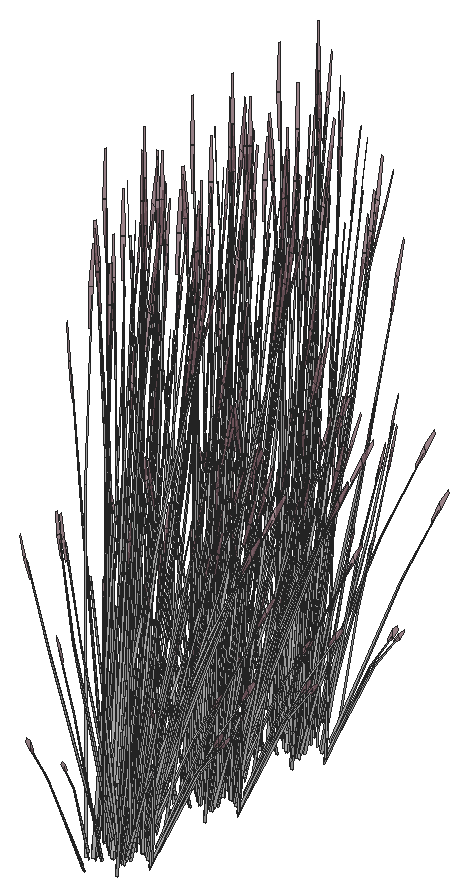
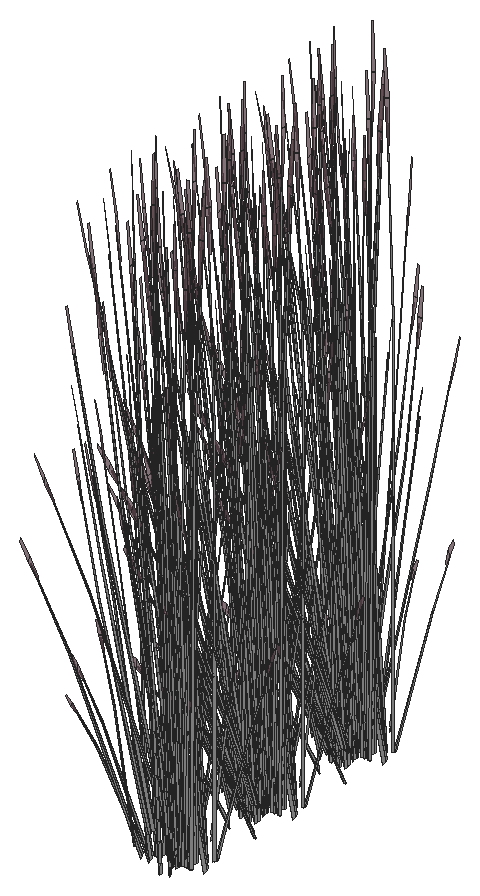
# SketchUp Ruby script. Lengths in inches.
U = 1.inch
M = Sketchup.active_model
def pt(a) = Geom::Point3d.new(a.map { |v| v * U })
def face(e, loops, mat)
  f = e.add_face(loops[0].map { |a| pt(a) })
  loops[1..].each { |l| e.add_face(l.map { |a| pt(a) }).erase! }
  f.material = f.back_material = mat if mat
  f
end
# faces: each face lists its corners as indices into pts; further lists are holes
def faces(e, pts, list, mat = nil) = list.each { |f| face(e, (f[0].is_a?(Array) ? f : [f]).map { |l| l.map { |i| pts[i] } }, mat) }
# xy, xz, yz: faces in a plane at the given z, y or x. An outline is a flat list of corners, or four numbers for a rectangle; further outlines are holes
def ring(l) = l.size == 4 ? [[l[0], l[1]], [l[2], l[1]], [l[2], l[3]], [l[0], l[3]]] : l.each_slice(2).to_a
def flat(e, list, mat, &to3) = list.each { |f| face(e, (f[0].is_a?(Array) ? f : [f]).map { |l| ring(l).map { |u, v| to3.(u, v) } }, mat) }
def xy(e, z, list, mat = nil) = flat(e, list, mat) { |x, y| [x, y, z] }
def xz(e, y, list, mat = nil) = flat(e, list, mat) { |x, z| [x, y, z] }
def yz(e, x, list, mat = nil) = flat(e, list, mat) { |y, z| [x, y, z] }
def lines(e, pts, list) = list.each { |a, b| e.add_line(pt(pts[a]), pt(pts[b])) }
# prism: a flat outline (further loops are holes) pulled along v
def prism(e, loops, v, mat = nil)
  f = face(e, loops, mat); d = Geom::Vector3d.new(v.map { |x| x * U })
  f.pushpull(f.normal.samedirection?(d) ? d.length : -d.length)
end
def box(e, o, s, mat = nil) = prism(e, [[o, [o[0] + s[0], o[1], o[2]], [o[0] + s[0], o[1] + s[1], o[2]], [o[0], o[1] + s[1], o[2]]]], [0, 0, s[2]], mat)
def at(x, y, z, deg = 0) = Geom::Transformation.translation(pt([x, y, z])) * Geom::Transformation.rotation(ORIGIN, Z_AXIS, deg.degrees)
def axes(o, x, y, z) = Geom::Transformation.new([*x, 0, *y, 0, *z, 0, *pt(o).to_a, 1])
def part(name) = M.definitions.add(name)
# library, detail: a bought-in or finely detailed component or shape, given as its bounding box
def library(name, o, s) = part(name).tap { |d| box(d.entities, o, s) }
def detail(e, o, s) = box(e.add_group.entities, o, s)
def put(e, d, t, mat = nil) = e.add_instance(d, t).tap { |i| i.material = mat if mat }
def group(e, t, mat = nil) = e.add_group.tap { |g| g.transformation = t; g.material = mat if mat }.entities
root = M.entities
M.materials.add("LightPink_Translucent").color = [144, 107, 117]
M.materials["LightPink_Translucent"].alpha = 0.75
M.materials.add("[_0053_Ivory_]").color = [200, 200, 200]
c1 = part("blade")
p = [[2.15,0.21,22],[0,0.17,0],[0.09,0.45,0],[2.18,0.31,22],[2.29,0.31,22],[0.38,0.45,0],
  [2.48,0.24,33],[2.49,0.24,33],[2.48,0.22,33]]
faces(c1.entities,p,[[0,1,2,3],[4,5,2,3],[6,3,4,7],[8,0,3,6]])
c2 = part("seeds")
p = [[0.3,-0.1,1.38],[-0.01,-0.03,1.59],[-0.01,-0.03,0.03],[0.14,-0.07,-0.07],[0.29,-0.03,3],[0.15,0.01,3.11]]
faces(c2.entities,p,[[0,1,2,3],[1,0,4,5]],"LightPink_Translucent")
c3 = part("blade with seeds")
put(c3.entities,c1,at(0,0,0))
put(c3.entities,c2,axes([2.4,0.25,30.99],[1.5799,-0.05474,1.17369],[-0.12525,1.92788,0.29478],[-0.07173,-0.02425,1.56792]))
put(root,c3,axes([680.98,251.57,36.24],[-0.17264,0.12729,1.43002],[-0.51703,-0.22279,-0.30754],[0.09584,-0.27707,0.61141]),"[_0053_Ivory_]")
put(root,c3,axes([679.7,250.88,35.15],[-0.10187,0.02266,1.76342],[-0.56336,-0.25503,-0.26939],[0.00945,-0.21273,0.30037]),"[_0053_Ivory_]")
put(root,c3,axes([681.4,252.52,38.63],[0.0158,-0.58168,-0.71045],[0.66548,0.03907,0.08574],[0.07023,-0.24643,1.00501]),"[_0053_Ivory_]")
put(root,c3,axes([680.25,251.58,38.18],[0.1831,-0.48359,-0.35414],[0.53419,0.14105,0.4572],[-0.04898,-0.1947,0.87481]),"[_0053_Ivory_]")
put(root,c3,axes([680.65,252.22,37.53],[-0.11309,0.21615,1.71376],[-0.47441,-0.44731,0.13857],[0.21402,-0.27879,0.73262]),"[_0053_Ivory_]")
put(root,c3,axes([680.35,250.5625,36.42],[0.07791,0.3667,1.1486],[-0.43222,-0.2031,0.84392],[0.04651,-0.18776,0.25299]),"[_0053_Ivory_]")
put(root,c3,axes([681.27,252.32,38.33],[-0.43478,-0.42253,-0.51099],[0.45929,-0.37004,-0.3958],[0.06615,-0.21468,0.97773]),"[_0053_Ivory_]")
put(root,c3,axes([681.68,252.17,38.18],[0.41095,-0.33109,-0.35414],[0.38901,0.37805,0.4572],[0.05919,-0.19208,0.87481]),"[_0053_Ivory_]")
put(root,c3,axes([682.19,251.97,35.15],[-0.0909,-0.04954,1.76342],[-0.2335,-0.55347,-0.26939],[0.15752,-0.1502,0.30037]),"[_0053_Ivory_]")
put(root,c3,axes([682.1875,253.53,38.63],[0.31725,-0.49618,-0.71045],[0.55593,0.35263,0.08574],[0.18942,-0.17977,1.00501]),"[_0053_Ivory_]")
put(root,c3,axes([678.76,252.08,36.03],[-0.37973,-0.63014,0],[0.6353,-0.35142,-0.51607],[0.14469,-0.08004,1.63711]),"[_0053_Ivory_]")
put(root,c3,axes([682.17,253.3,38.33],[-0.15602,-0.5742,-0.51099],[0.59087,-0.10045,-0.3958],[0.16933,-0.15423,0.97773]),"[_0053_Ivory_]")
put(root,c3,axes([679.27,251.99,35.67],[0.56842,-0.31443,-0.49651],[0.33976,0.56381,0],[0.12946,-0.07161,1.57504]),"[_0053_Ivory_]")
put(root,c3,axes([682.65,253.07,36.24],[-0.21697,-0.01863,1.43002],[-0.22228,-0.49966,-0.30754],[0.26655,-0.14135,0.61141]),"[_0053_Ivory_]")
put(root,c3,axes([679.95,253.28,35.71],[0.40909,-0.47266,-0.62353],[0.50819,0.4286,-0.16365],[0.16393,-0.11791,1.37633]),"[_0053_Ivory_]")
put(root,c3,axes([682.9,252.15,36.42],[-0.2023,0.32011,1.1486],[-0.17388,-0.43009,0.84392],[0.16708,-0.10777,0.25299]),"[_0053_Ivory_]")
put(root,c3,axes([682.61,253.36,38.18],[0.52868,-0.08987,-0.35414],[0.1396,0.51376,0.4572],[0.1515,-0.13799,0.87481]),"[_0053_Ivory_]")
put(root,c3,axes([679.24,254.1,35.86],[0.29468,-0.56664,-0.44739],[0.61229,0.27271,0.21531],[0,-0.13062,1.43643]),"[_0053_Ivory_]")
put(root,c3,axes([679.5,253.82,36.32],[-0.07077,-0.71755,-0.29095],[0.73712,-0.04339,-0.50002],[0.1298,-0.09558,1.59708]),"[_0053_Ivory_]")
put(root,c3,axes([679.41,252.23,35.68],[0.56663,0.1556,-0.30978],[-0.14267,0.54795,0.30978],[0.11423,-0.06319,1.38974]),"[_0053_Ivory_]")
put(root,c3,axes([679.6,254.39,36.09],[0.68433,0.30479,0.24065],[-0.32934,0.63331,0.50002],[0,-0.14599,1.60543]),"[_0053_Ivory_]")
put(root,c3,axes([679.38,253.96,36.37],[-0.65953,0.03882,0.44739],[-0.05964,-0.64439,-0.21531],[0.11807,-0.06531,1.43643]),"[_0053_Ivory_]")
put(root,c3,axes([682.45,254.57,38.33],[0.16454,-0.57202,-0.51099],[0.56413,0.19607,-0.3958],[0.22713,-0.05245,0.97773]),"[_0053_Ivory_]")
put(root,c3,axes([681.55,252.24,36.03],[0.37973,-0.63014,0],[0.6353,0.35142,-0.51607],[0.14469,0.08004,1.63711]),"[_0053_Ivory_]")
put(root,c3,axes([679.36,254.19,36.01],[0.26406,0.70318,0.45755],[-0.7545,0.24452,0.17955],[0.00922,-0.12921,1.58856]),"[_0053_Ivory_]")
put(root,c3,axes([683.05,254.73,35.64],[-0.39118,0.07547,1.41583],[-0.06226,-0.6007,0.08104],[0.27398,-0.09092,0.80566]),"[_0053_Ivory_]")
put(root,c3,axes([683.76,254.2,35.91],[-0.37654,-0.40212,-0.06488],[0.4124,-0.36845,-0.29416],[0.11685,-0.02594,0.97024]),"[_0053_Ivory_]")
put(root,c3,axes([680.31,254.25,35.86],[0,-0.72763,0],[0.75945,0,0],[0,0,1.79456]),"[_0053_Ivory_]")
put(root,c3,axes([681.23,252.57,36.13],[-0.56842,-0.31443,0.49651],[0.33976,-0.56381,0],[0.12946,0.07161,1.57504]),"[_0053_Ivory_]")
put(root,c3,axes([682.34,254.78,38.63],[0.53369,-0.27773,-0.71045],[0.29743,0.5717,0.08574],[0.25786,-0.06494,1.00501]),"[_0053_Ivory_]")
put(root,c3,axes([679.95,253.79,36.01],[-0.50358,0.57069,0.45755],[-0.59827,-0.50377,0.17955],[0.1214,-0.05695,1.58856]),"[_0053_Ivory_]")
put(root,c3,axes([679.07,252.85,36.13],[-0.17545,0.62497,0.17642],[-0.64204,-0.17686,0.35086],[0.11091,-0.00304,1.60407]),"[_0053_Ivory_]")
put(root,c3,axes([678.81,253.36,35.25],[-0.59782,0.25177,1.28929],[-0.19028,-0.72239,0.50096],[0.36709,0.01202,1.46642]),"[_0053_Ivory_]")
put(root,c3,axes([680.41,253.55,36.27],[0.11717,-0.56122,0.1448],[0.57245,0.09742,-0.41347],[0.10418,0.05763,1.26744]),"[_0053_Ivory_]")
put(root,c3,axes([683.48,254.34,35.15],[-0.03174,-0.09547,1.76342],[0.22015,-0.55846,-0.26939],[0.22208,-0.00803,0.30037]),"[_0053_Ivory_]")
put(root,c3,axes([680.17,253.7,36.37],[-0.36485,-0.52782,0.44739],[0.55265,-0.37168,-0.21531],[0.11807,0.06531,1.43643]),"[_0053_Ivory_]")
put(root,c3,axes([680.35,253.73,36.32],[0.61322,-0.4175,-0.29095],[0.40778,0.58992,-0.50002],[0.1513,0.05991,1.59708]),"[_0053_Ivory_]")
put(root,c3,axes([682.79,254.83,38.18],[0.50475,0.17543,-0.35414],[-0.14722,0.5118,0.4572],[0.20322,-0.04693,0.87481]),"[_0053_Ivory_]")
put(root,c3,axes([681.9,252.62,35.67],[0.56842,0.31443,-0.49651],[-0.33976,0.56381,0],[0.12946,0.07161,1.57504]),"[_0053_Ivory_]")
put(root,c3,axes([680.82,254.42,35.86],[0.67951,0,0],[0,0.65103,0],[0,0,1.78407]),"[_0053_Ivory_]")
put(root,c3,axes([681.01,252.89,36.13],[-0.65264,0.16691,0.17642],[-0.16115,-0.62115,0.35086],[0.05821,0.0905,1.60407]),"[_0053_Ivory_]")
put(root,c3,axes([681.42,254.2,37.53],[-0.25192,0.01424,1.71376],[0.16712,-0.61729,0.13857],[0.35901,0.03818,0.73262]),"[_0053_Ivory_]")
put(root,c3,axes([681.74,252.86,35.68],[0.14267,0.54795,-0.30978],[-0.56663,0.1556,0.30978],[0.11423,0.06319,1.38974]),"[_0053_Ivory_]")
put(root,c3,axes([680.6,254.08,36.03],[-0.76764,-0.13249,0.49198],[0.15622,-0.74829,0.19306],[0.11218,0.07226,1.70813]),"[_0053_Ivory_]")
put(root,c3,axes([679.99,255.93,35.86],[-0.19817,-0.54216,0],[0.56587,-0.18986,0],[0,0,1.54371]),"[_0053_Ivory_]")
put(root,c3,axes([680.73,255.86,35.84],[0.63764,-0.21337,-0.19198],[0.22406,0.61462,0.00008],[0.07038,-0.02358,1.73897]),"[_0053_Ivory_]")
put(root,c3,axes([680.81,254.69,35.87],[0.42396,0.40619,0],[-0.42396,0.40619,0],[0,0,1.69266]),"[_0053_Ivory_]")
put(root,c3,axes([681.95,254.52,36.13],[-0.47719,-0.45806,0.17642],[0.48088,-0.44429,0.35086],[-0.0527,0.09355,1.60407]),"[_0053_Ivory_]")
put(root,c3,axes([681.07,253.83,35.71],[0.63179,0.1031,-0.62353],[-0.13332,0.63596,-0.16365],[0.18854,0.07706,1.37633]),"[_0053_Ivory_]")
put(root,c3,axes([683.86,254.9375,36.42],[-0.37526,0.10382,1.1486],[0.17664,-0.42906,0.84392],[0.19907,0.02936,0.25299]),"[_0053_Ivory_]")
put(root,c3,axes([680.8,254.22,36.37],[0.29468,-0.56664,0.44739],[0.61229,0.27271,-0.21531],[0,0.13062,1.43643]),"[_0053_Ivory_]")
put(root,c3,axes([680.6875,254.54,35.95],[0,0.72727,-0.05637],[-0.75945,0,0],[0,0.02286,1.79368]),"[_0053_Ivory_]")
put(root,c3,axes([680.74,254.03,35.86],[0.36485,0.52782,-0.44739],[-0.55265,0.37168,0.21531],[0.11807,0.06531,1.43643]),"[_0053_Ivory_]")
put(root,c3,axes([683.21,256.26,37.58],[-0.11624,-0.52862,-0.03492],[0.54943,-0.12153,-0.15832],[0.11473,0.03351,0.52218]),"[_0053_Ivory_]")
put(root,c3,axes([682.35,254.54,36.13],[0,-0.62885,0.49651],[0.67951,0,0],[0,0.14322,1.57504]),"[_0053_Ivory_]")
put(root,c3,axes([681.06,254.35,36.27],[0.56587,-0.18339,0.1448],[0.19817,0.52368,-0.41347],[0,0.11525,1.26744]),"[_0053_Ivory_]")
put(root,c3,axes([683.16,255.625,36.24],[-0.14627,-0.15466,1.43002],[0.19032,-0.51164,-0.30754],[0.29594,0.06931,0.61141]),"[_0053_Ivory_]")
put(root,c3,axes([680.55,256.1875,35.86],[0.61229,0.28233,0],[-0.29468,0.58663,0],[0,0,1.74954]),"[_0053_Ivory_]")
put(root,c3,axes([681.82,255.9375,38.63],[0.60713,0.01514,-0.71045],[-0.04078,0.63759,0.08574],[0.25721,0.06729,1.00501]),"[_0053_Ivory_]")
put(root,c3,axes([681.13,256.45,36.13],[0.56842,-0.31443,0.49651],[0.33976,0.56381,0],[-0.12946,0.07161,1.57504]),"[_0053_Ivory_]")
put(root,c3,axes([680.32,255.95,35.94],[0.26406,0.72244,-0.06012],[-0.7545,0.25315,0],[0.00922,0.02523,1.72173]),"[_0053_Ivory_]")
put(root,c3,axes([682.81,254.64,36.03],[0.75945,0,0],[0,0.70283,-0.51607],[0,0.16007,1.63711]),"[_0053_Ivory_]")
put(root,c3,axes([682.51,255,35.85],[-0.75908,-0.00503,-0.04976],[0,-0.70283,0.49943],[-0.02386,0.16,1.58352]),"[_0053_Ivory_]")
put(root,c3,axes([680.86,254.39,36.32],[0.68399,0.30005,-0.29095],[-0.32934,0.63331,-0.50002],[0.0215,0.15549,1.59708]),"[_0053_Ivory_]")
put(root,c3,axes([680.98,262.72,36.24],[-0.17264,0.12729,1.43002],[-0.51703,-0.22279,-0.30754],[0.09584,-0.27707,0.61141]),"[_0053_Ivory_]")
put(root,c3,axes([682.18,256.2,38.18],[0.34557,0.39372,-0.35414],[-0.39459,0.37271,0.4572],[0.20048,0.05671,0.87481]),"[_0053_Ivory_]")
put(root,c3,axes([682.35,255.11,35.68],[-0.42396,0.39235,-0.30978],[-0.42396,-0.39235,0.30978],[0,0.12637,1.38974]),"[_0053_Ivory_]")
put(root,c3,axes([680.79,254.86,35.86],[-0.29468,0.56664,-0.44739],[-0.61229,-0.27271,0.21531],[0,0.13062,1.43643]),"[_0053_Ivory_]")
put(root,c3,axes([679.7,262.03,35.15],[-0.10187,0.02266,1.76342],[-0.56336,-0.25503,-0.26939],[0.00945,-0.21273,0.30037]),"[_0053_Ivory_]")
put(root,c3,axes([681.4,263.67,38.63],[0.0158,-0.58168,-0.71045],[0.66548,0.03907,0.08574],[0.07023,-0.24643,1.00501]),"[_0053_Ivory_]")
put(root,c3,axes([680.25,262.73,38.18],[0.1831,-0.48359,-0.35414],[0.53419,0.14105,0.4572],[-0.04898,-0.1947,0.87481]),"[_0053_Ivory_]")
put(root,c3,axes([680.65,263.37,37.53],[-0.11309,0.21615,1.71376],[-0.47441,-0.44731,0.13857],[0.21402,-0.27879,0.73262]),"[_0053_Ivory_]")
put(root,c3,axes([682.64,255.12,35.67],[0,0.62885,-0.49651],[-0.67951,0,0],[0,0.14322,1.57504]),"[_0053_Ivory_]")
put(root,c3,axes([680.94,255.19,37.53],[-0.2256,-0.10835,1.71376],[0.46687,-0.45453,0.13857],[0.29098,0.20505,0.73262]),"[_0053_Ivory_]")
put(root,c3,axes([680.35,261.71,36.42],[0.07791,0.3667,1.1486],[-0.43222,-0.2031,0.84392],[0.04651,-0.18776,0.25299]),"[_0053_Ivory_]")
put(root,c3,axes([681.27,263.47,38.33],[-0.43478,-0.42253,-0.51099],[0.45929,-0.37004,-0.3958],[0.06615,-0.21468,0.97773]),"[_0053_Ivory_]")
put(root,c3,axes([681.78,256.42,36.42],[-0.34197,-0.18082,1.1486],[0.44156,-0.18372,0.84392],[0.1191,0.15563,0.25299]),"[_0053_Ivory_]")
put(root,c3,axes([681.87,257.1,35.15],[0.04425,-0.09079,1.76342],[0.55709,-0.26738,-0.26939],[0.16889,0.13839,0.30037]),"[_0053_Ivory_]")
put(root,c3,axes([681.14,255.03,35.75],[0.2227,0.57576,-0.69212],[-0.64151,0.20736,-0.18165],[0.02462,0.19497,1.52773]),"[_0053_Ivory_]")
put(root,c3,axes([681.68,263.32,38.18],[0.41095,-0.33109,-0.35414],[0.38901,0.37805,0.4572],[0.05919,-0.19208,0.87481]),"[_0053_Ivory_]")
put(root,c3,axes([681,256.67,38.33],[0.59932,-0.14948,-0.51099],[0.10484,0.56611,-0.3958],[0.16097,0.16223,0.97773]),"[_0053_Ivory_]")
put(root,c3,axes([681.83,257.25,36.32],[-0.38947,-0.01972,1.0506],[0.25721,-0.41888,0.58006],[0.15386,0.14882,0.8241]),"[_0053_Ivory_]")
put(root,c3,axes([682.19,263.12,35.15],[-0.0909,-0.04954,1.76342],[-0.2335,-0.55347,-0.26939],[0.15752,-0.1502,0.30037]),"[_0053_Ivory_]")
put(root,c3,axes([680.56,256.23,36.24],[0.01072,-0.20846,1.43002],[0.51218,-0.23285,-0.30754],[0.15811,0.2495,0.61141]),"[_0053_Ivory_]")
put(root,c3,axes([682.1875,264.68,38.63],[0.31725,-0.49618,-0.71045],[0.55593,0.35263,0.08574],[0.18942,-0.17977,1.00501]),"[_0053_Ivory_]")
put(root,c3,axes([678.76,263.23,36.03],[-0.37973,-0.63014,0],[0.6353,-0.35142,-0.51607],[0.14469,-0.08004,1.63711]),"[_0053_Ivory_]")
put(root,c3,axes([682.17,264.44,38.33],[-0.15602,-0.5742,-0.51099],[0.59087,-0.10045,-0.3958],[0.16933,-0.15423,0.97773]),"[_0053_Ivory_]")
put(root,c3,axes([679.27,257.08,35.15],[0.09829,-0.03422,1.76342],[0.59126,0.18834,-0.26939],[0.01729,0.21228,0.30037]),"[_0053_Ivory_]")
put(root,c3,axes([679.67,256.94,38.33],[0.59704,0.15764,-0.51099],[-0.20464,0.54049,-0.3958],[0.05475,0.21761,0.97773]),"[_0053_Ivory_]")
put(root,c3,axes([680.01,255.82,37.53],[-0.13883,-0.2019,1.71376],[0.64153,-0.16998,0.13857],[0.14499,0.31697,0.73262]),"[_0053_Ivory_]")
put(root,c3,axes([679.4,257.27,38.18],[-0.1831,0.48359,-0.35414],[-0.53419,-0.14105,0.4572],[0.04898,0.1947,0.87481]),"[_0053_Ivory_]")
put(root,c3,axes([679.27,263.13,35.67],[0.56842,-0.31443,-0.49651],[0.33976,0.56381,0],[0.12946,-0.07161,1.57504]),"[_0053_Ivory_]")
put(root,c3,axes([682.65,264.22,36.24],[-0.21697,-0.01863,1.43002],[-0.22228,-0.49966,-0.30754],[0.26655,-0.14135,0.61141]),"[_0053_Ivory_]")
put(root,c3,axes([679.95,264.42,35.71],[0.40909,-0.47266,-0.62353],[0.50819,0.4286,-0.16365],[0.16393,-0.11791,1.37633]),"[_0053_Ivory_]")
put(root,c3,axes([682.9,263.3,36.42],[-0.2023,0.32011,1.1486],[-0.17388,-0.43009,0.84392],[0.16708,-0.10777,0.25299]),"[_0053_Ivory_]")
put(root,c3,axes([682.61,264.51,38.18],[0.52868,-0.08987,-0.35414],[0.1396,0.51376,0.4572],[0.1515,-0.13799,0.87481]),"[_0053_Ivory_]")
put(root,c3,axes([679.46,256.83,38.63],[0.28988,0.51132,-0.71045],[-0.59671,0.28496,0.08574],[0.06778,0.24706,1.00501]),"[_0053_Ivory_]")
put(root,c3,axes([679.24,265.25,35.86],[0.29468,-0.56664,-0.44739],[0.61229,0.27271,0.21531],[0,-0.13062,1.43643]),"[_0053_Ivory_]")
put(root,c3,axes([679.5,264.97,36.32],[-0.07077,-0.71755,-0.29095],[0.73712,-0.04339,-0.50002],[0.1298,-0.09558,1.59708]),"[_0053_Ivory_]")
put(root,c3,axes([679.41,263.38,35.68],[0.56663,0.1556,-0.30978],[-0.14267,0.54795,0.30978],[0.11423,-0.06319,1.38974]),"[_0053_Ivory_]")
put(root,c3,axes([679.6,265.53,36.09],[0.68433,0.30479,0.24065],[-0.32934,0.63331,0.50002],[0,-0.14599,1.60543]),"[_0053_Ivory_]")
put(root,c3,axes([679.38,265.11,36.37],[-0.65953,0.03882,0.44739],[-0.05964,-0.64439,-0.21531],[0.11807,-0.06531,1.43643]),"[_0053_Ivory_]")
put(root,c3,axes([682.45,265.72,38.33],[0.16454,-0.57202,-0.51099],[0.56413,0.19607,-0.3958],[0.22713,-0.05245,0.97773]),"[_0053_Ivory_]")
put(root,c3,axes([681.55,263.39,36.03],[0.37973,-0.63014,0],[0.6353,0.35142,-0.51607],[0.14469,0.08004,1.63711]),"[_0053_Ivory_]")
put(root,c3,axes([679.36,265.34,36.01],[0.26406,0.70318,0.45755],[-0.7545,0.24452,0.17955],[0.00922,-0.12921,1.58856]),"[_0053_Ivory_]")
put(root,c3,axes([683.05,265.88,35.64],[-0.39118,0.07547,1.41583],[-0.06226,-0.6007,0.08104],[0.27398,-0.09092,0.80566]),"[_0053_Ivory_]")
put(root,c3,axes([683.76,265.35,35.91],[-0.37654,-0.40212,-0.06488],[0.4124,-0.36845,-0.29416],[0.11685,-0.02594,0.97024]),"[_0053_Ivory_]")
put(root,c3,axes([680.31,265.4,35.86],[0,-0.72763,0],[0.75945,0,0],[0,0,1.79456]),"[_0053_Ivory_]")
put(root,c3,axes([681.23,263.72,36.13],[-0.56842,-0.31443,0.49651],[0.33976,-0.56381,0],[0.12946,0.07161,1.57504]),"[_0053_Ivory_]")
put(root,c3,axes([682.34,265.93,38.63],[0.53369,-0.27773,-0.71045],[0.29743,0.5717,0.08574],[0.25786,-0.06494,1.00501]),"[_0053_Ivory_]")
put(root,c3,axes([679.95,264.94,36.01],[-0.50358,0.57069,0.45755],[-0.59827,-0.50377,0.17955],[0.1214,-0.05695,1.58856]),"[_0053_Ivory_]")
put(root,c3,axes([679.07,264,36.13],[-0.17545,0.62497,0.17642],[-0.64204,-0.17686,0.35086],[0.11091,-0.00304,1.60407]),"[_0053_Ivory_]")
put(root,c3,axes([678.81,264.51,35.25],[-0.59782,0.25177,1.28929],[-0.19028,-0.72239,0.50096],[0.36709,0.01202,1.46642]),"[_0053_Ivory_]")
put(root,c3,axes([680.41,264.7,36.27],[0.11717,-0.56122,0.1448],[0.57245,0.09742,-0.41347],[0.10418,0.05763,1.26744]),"[_0053_Ivory_]")
put(root,c3,axes([683.48,265.49,35.15],[-0.03174,-0.09547,1.76342],[0.22015,-0.55846,-0.26939],[0.22208,-0.00803,0.30037]),"[_0053_Ivory_]")
put(root,c3,axes([680.17,264.85,36.37],[-0.36485,-0.52782,0.44739],[0.55265,-0.37168,-0.21531],[0.11807,0.06531,1.43643]),"[_0053_Ivory_]")
put(root,c3,axes([680.35,264.88,36.32],[0.61322,-0.4175,-0.29095],[0.40778,0.58992,-0.50002],[0.1513,0.05991,1.59708]),"[_0053_Ivory_]")
put(root,c3,axes([682.79,265.98,38.18],[0.50475,0.17543,-0.35414],[-0.14722,0.5118,0.4572],[0.20322,-0.04693,0.87481]),"[_0053_Ivory_]")
put(root,c3,axes([681.9,263.77,35.67],[0.56842,0.31443,-0.49651],[-0.33976,0.56381,0],[0.12946,0.07161,1.57504]),"[_0053_Ivory_]")
put(root,c3,axes([680.82,265.5625,35.86],[0.67951,0,0],[0,0.65103,0],[0,0,1.78407]),"[_0053_Ivory_]")
put(root,c3,axes([681.01,264.04,36.13],[-0.65264,0.16691,0.17642],[-0.16115,-0.62115,0.35086],[0.05821,0.0905,1.60407]),"[_0053_Ivory_]")
put(root,c3,axes([681.42,265.35,37.53],[-0.25192,0.01424,1.71376],[0.16712,-0.61729,0.13857],[0.35901,0.03818,0.73262]),"[_0053_Ivory_]")
put(root,c3,axes([681.74,264.01,35.68],[0.14267,0.54795,-0.30978],[-0.56663,0.1556,0.30978],[0.11423,0.06319,1.38974]),"[_0053_Ivory_]")
put(root,c3,axes([680.6,265.23,36.03],[-0.76764,-0.13249,0.49198],[0.15622,-0.74829,0.19306],[0.11218,0.07226,1.70813]),"[_0053_Ivory_]")
put(root,c3,axes([679.99,267.08,35.86],[-0.19817,-0.54216,0],[0.56587,-0.18986,0],[0,0,1.54371]),"[_0053_Ivory_]")
put(root,c3,axes([680.73,267,35.84],[0.63764,-0.21337,-0.19198],[0.22406,0.61462,0.00008],[0.07038,-0.02358,1.73897]),"[_0053_Ivory_]")
put(root,c3,axes([680.81,265.84,35.87],[0.42396,0.40619,0],[-0.42396,0.40619,0],[0,0,1.69266]),"[_0053_Ivory_]")
put(root,c3,axes([681.95,265.67,36.13],[-0.47719,-0.45806,0.17642],[0.48088,-0.44429,0.35086],[-0.0527,0.09355,1.60407]),"[_0053_Ivory_]")
put(root,c3,axes([681.07,264.97,35.71],[0.63179,0.1031,-0.62353],[-0.13332,0.63596,-0.16365],[0.18854,0.07706,1.37633]),"[_0053_Ivory_]")
put(root,c3,axes([683.86,266.09,36.42],[-0.37526,0.10382,1.1486],[0.17664,-0.42906,0.84392],[0.19907,0.02936,0.25299]),"[_0053_Ivory_]")
put(root,c3,axes([680.8,265.37,36.37],[0.29468,-0.56664,0.44739],[0.61229,0.27271,-0.21531],[0,0.13062,1.43643]),"[_0053_Ivory_]")
put(root,c3,axes([680.6875,265.69,35.95],[0,0.72727,-0.05637],[-0.75945,0,0],[0,0.02286,1.79368]),"[_0053_Ivory_]")
put(root,c3,axes([680.74,265.18,35.86],[0.36485,0.52782,-0.44739],[-0.55265,0.37168,0.21531],[0.11807,0.06531,1.43643]),"[_0053_Ivory_]")
put(root,c3,axes([683.21,267.41,37.58],[-0.11624,-0.52862,-0.03492],[0.54943,-0.12153,-0.15832],[0.11473,0.03351,0.52218]),"[_0053_Ivory_]")
put(root,c3,axes([682.35,265.68,36.13],[0,-0.62885,0.49651],[0.67951,0,0],[0,0.14322,1.57504]),"[_0053_Ivory_]")
put(root,c3,axes([681.06,265.5,36.27],[0.56587,-0.18339,0.1448],[0.19817,0.52368,-0.41347],[0,0.11525,1.26744]),"[_0053_Ivory_]")
put(root,c3,axes([683.16,266.77,36.24],[-0.14627,-0.15466,1.43002],[0.19032,-0.51164,-0.30754],[0.29594,0.06931,0.61141]),"[_0053_Ivory_]")
put(root,c3,axes([680.55,267.34,35.86],[0.61229,0.28233,0],[-0.29468,0.58663,0],[0,0,1.74954]),"[_0053_Ivory_]")
put(root,c3,axes([681.82,267.08,38.63],[0.60713,0.01514,-0.71045],[-0.04078,0.63759,0.08574],[0.25721,0.06729,1.00501]),"[_0053_Ivory_]")
put(root,c3,axes([681.13,267.6,36.13],[0.56842,-0.31443,0.49651],[0.33976,0.56381,0],[-0.12946,0.07161,1.57504]),"[_0053_Ivory_]")
put(root,c3,axes([680.32,267.1,35.94],[0.26406,0.72244,-0.06012],[-0.7545,0.25315,0],[0.00922,0.02523,1.72173]),"[_0053_Ivory_]")
put(root,c3,axes([682.81,265.79,36.03],[0.75945,0,0],[0,0.70283,-0.51607],[0,0.16007,1.63711]),"[_0053_Ivory_]")
put(root,c3,axes([680.98,273.71,36.24],[-0.17264,0.12729,1.43002],[-0.51703,-0.22279,-0.30754],[0.09584,-0.27707,0.61141]),"[_0053_Ivory_]")
put(root,c3,axes([682.51,266.15,35.85],[-0.75908,-0.00503,-0.04976],[0,-0.70283,0.49943],[-0.02386,0.16,1.58352]),"[_0053_Ivory_]")
put(root,c3,axes([680.86,265.54,36.32],[0.68399,0.30005,-0.29095],[-0.32934,0.63331,-0.50002],[0.0215,0.15549,1.59708]),"[_0053_Ivory_]")
put(root,c3,axes([682.18,267.35,38.18],[0.34557,0.39372,-0.35414],[-0.39459,0.37271,0.4572],[0.20048,0.05671,0.87481]),"[_0053_Ivory_]")
put(root,c3,axes([682.35,266.25,35.68],[-0.42396,0.39235,-0.30978],[-0.42396,-0.39235,0.30978],[0,0.12637,1.38974]),"[_0053_Ivory_]")
put(root,c3,axes([680.79,266.01,35.86],[-0.29468,0.56664,-0.44739],[-0.61229,-0.27271,0.21531],[0,0.13062,1.43643]),"[_0053_Ivory_]")
put(root,c3,axes([679.7,273.02,35.15],[-0.10187,0.02266,1.76342],[-0.56336,-0.25503,-0.26939],[0.00945,-0.21273,0.30037]),"[_0053_Ivory_]")
put(root,c3,axes([681.4,274.66,38.63],[0.0158,-0.58168,-0.71045],[0.66548,0.03907,0.08574],[0.07023,-0.24643,1.00501]),"[_0053_Ivory_]")
put(root,c3,axes([680.25,273.72,38.18],[0.1831,-0.48359,-0.35414],[0.53419,0.14105,0.4572],[-0.04898,-0.1947,0.87481]),"[_0053_Ivory_]")
put(root,c3,axes([680.65,274.36,37.53],[-0.11309,0.21615,1.71376],[-0.47441,-0.44731,0.13857],[0.21402,-0.27879,0.73262]),"[_0053_Ivory_]")
put(root,c3,axes([682.64,266.27,35.67],[0,0.62885,-0.49651],[-0.67951,0,0],[0,0.14322,1.57504]),"[_0053_Ivory_]")
put(root,c3,axes([680.35,272.7,36.42],[0.07791,0.3667,1.1486],[-0.43222,-0.2031,0.84392],[0.04651,-0.18776,0.25299]),"[_0053_Ivory_]")
put(root,c3,axes([680.94,266.34,37.53],[-0.2256,-0.10835,1.71376],[0.46687,-0.45453,0.13857],[0.29098,0.20505,0.73262]),"[_0053_Ivory_]")
put(root,c3,axes([681.27,274.46,38.33],[-0.43478,-0.42253,-0.51099],[0.45929,-0.37004,-0.3958],[0.06615,-0.21468,0.97773]),"[_0053_Ivory_]")
put(root,c3,axes([681.78,267.57,36.42],[-0.34197,-0.18082,1.1486],[0.44156,-0.18372,0.84392],[0.1191,0.15563,0.25299]),"[_0053_Ivory_]")
put(root,c3,axes([681.68,274.31,38.18],[0.41095,-0.33109,-0.35414],[0.38901,0.37805,0.4572],[0.05919,-0.19208,0.87481]),"[_0053_Ivory_]")
put(root,c3,axes([681.87,268.24,35.15],[0.04425,-0.09079,1.76342],[0.55709,-0.26738,-0.26939],[0.16889,0.13839,0.30037]),"[_0053_Ivory_]")
put(root,c3,axes([681.14,266.18,35.75],[0.2227,0.57576,-0.69212],[-0.64151,0.20736,-0.18165],[0.02462,0.19497,1.52773]),"[_0053_Ivory_]")
put(root,c3,axes([681,267.82,38.33],[0.59932,-0.14948,-0.51099],[0.10484,0.56611,-0.3958],[0.16097,0.16223,0.97773]),"[_0053_Ivory_]")
put(root,c3,axes([681.83,268.4,36.32],[-0.38947,-0.01972,1.0506],[0.25721,-0.41888,0.58006],[0.15386,0.14882,0.8241]),"[_0053_Ivory_]")
put(root,c3,axes([682.19,274.11,35.15],[-0.0909,-0.04954,1.76342],[-0.2335,-0.55347,-0.26939],[0.15752,-0.1502,0.30037]),"[_0053_Ivory_]")
put(root,c3,axes([680.56,267.38,36.24],[0.01072,-0.20846,1.43002],[0.51218,-0.23285,-0.30754],[0.15811,0.2495,0.61141]),"[_0053_Ivory_]")
put(root,c3,axes([682.1875,275.67,38.63],[0.31725,-0.49618,-0.71045],[0.55593,0.35263,0.08574],[0.18942,-0.17977,1.00501]),"[_0053_Ivory_]")
put(root,c3,axes([678.76,274.22,36.03],[-0.37973,-0.63014,0],[0.6353,-0.35142,-0.51607],[0.14469,-0.08004,1.63711]),"[_0053_Ivory_]")
put(root,c3,axes([682.17,275.4375,38.33],[-0.15602,-0.5742,-0.51099],[0.59087,-0.10045,-0.3958],[0.16933,-0.15423,0.97773]),"[_0053_Ivory_]")
put(root,c3,axes([679.27,268.22,35.15],[0.09829,-0.03422,1.76342],[0.59126,0.18834,-0.26939],[0.01729,0.21228,0.30037]),"[_0053_Ivory_]")
put(root,c3,axes([679.67,268.08,38.33],[0.59704,0.15764,-0.51099],[-0.20464,0.54049,-0.3958],[0.05475,0.21761,0.97773]),"[_0053_Ivory_]")
put(root,c3,axes([680.01,266.97,37.53],[-0.13883,-0.2019,1.71376],[0.64153,-0.16998,0.13857],[0.14499,0.31697,0.73262]),"[_0053_Ivory_]")
put(root,c3,axes([679.27,274.125,35.67],[0.56842,-0.31443,-0.49651],[0.33976,0.56381,0],[0.12946,-0.07161,1.57504]),"[_0053_Ivory_]")
put(root,c3,axes([682.65,275.21,36.24],[-0.21697,-0.01863,1.43002],[-0.22228,-0.49966,-0.30754],[0.26655,-0.14135,0.61141]),"[_0053_Ivory_]")
put(root,c3,axes([679.4,268.42,38.18],[-0.1831,0.48359,-0.35414],[-0.53419,-0.14105,0.4572],[0.04898,0.1947,0.87481]),"[_0053_Ivory_]")
put(root,c3,axes([679.95,275.42,35.71],[0.40909,-0.47266,-0.62353],[0.50819,0.4286,-0.16365],[0.16393,-0.11791,1.37633]),"[_0053_Ivory_]")
put(root,c3,axes([682.9,274.29,36.42],[-0.2023,0.32011,1.1486],[-0.17388,-0.43009,0.84392],[0.16708,-0.10777,0.25299]),"[_0053_Ivory_]")
put(root,c3,axes([682.61,275.5,38.18],[0.52868,-0.08987,-0.35414],[0.1396,0.51376,0.4572],[0.1515,-0.13799,0.87481]),"[_0053_Ivory_]")
put(root,c3,axes([679.24,276.24,35.86],[0.29468,-0.56664,-0.44739],[0.61229,0.27271,0.21531],[0,-0.13062,1.43643]),"[_0053_Ivory_]")
put(root,c3,axes([679.5,275.96,36.32],[-0.07077,-0.71755,-0.29095],[0.73712,-0.04339,-0.50002],[0.1298,-0.09558,1.59708]),"[_0053_Ivory_]")
put(root,c3,axes([679.46,267.98,38.63],[0.28988,0.51132,-0.71045],[-0.59671,0.28496,0.08574],[0.06778,0.24706,1.00501]),"[_0053_Ivory_]")
put(root,c3,axes([679.41,274.375,35.68],[0.56663,0.1556,-0.30978],[-0.14267,0.54795,0.30978],[0.11423,-0.06319,1.38974]),"[_0053_Ivory_]")
put(root,c3,axes([679.6,276.53,36.09],[0.68433,0.30479,0.24065],[-0.32934,0.63331,0.50002],[0,-0.14599,1.60543]),"[_0053_Ivory_]")
put(root,c3,axes([679.38,276.1,36.37],[-0.65953,0.03882,0.44739],[-0.05964,-0.64439,-0.21531],[0.11807,-0.06531,1.43643]),"[_0053_Ivory_]")
put(root,c3,axes([682.45,276.71,38.33],[0.16454,-0.57202,-0.51099],[0.56413,0.19607,-0.3958],[0.22713,-0.05245,0.97773]),"[_0053_Ivory_]")
put(root,c3,axes([681.55,274.38,36.03],[0.37973,-0.63014,0],[0.6353,0.35142,-0.51607],[0.14469,0.08004,1.63711]),"[_0053_Ivory_]")
put(root,c3,axes([679.36,276.33,36.01],[0.26406,0.70318,0.45755],[-0.7545,0.24452,0.17955],[0.00922,-0.12921,1.58856]),"[_0053_Ivory_]")
put(root,c3,axes([683.05,276.87,35.64],[-0.39118,0.07547,1.41583],[-0.06226,-0.6007,0.08104],[0.27398,-0.09092,0.80566]),"[_0053_Ivory_]")
put(root,c3,axes([683.76,276.34,35.91],[-0.37654,-0.40212,-0.06488],[0.4124,-0.36845,-0.29416],[0.11685,-0.02594,0.97024]),"[_0053_Ivory_]")
put(root,c3,axes([680.31,276.39,35.86],[0,-0.72763,0],[0.75945,0,0],[0,0,1.79456]),"[_0053_Ivory_]")
put(root,c3,axes([681.23,274.71,36.13],[-0.56842,-0.31443,0.49651],[0.33976,-0.56381,0],[0.12946,0.07161,1.57504]),"[_0053_Ivory_]")
put(root,c3,axes([682.34,276.92,38.63],[0.53369,-0.27773,-0.71045],[0.29743,0.5717,0.08574],[0.25786,-0.06494,1.00501]),"[_0053_Ivory_]")
put(root,c3,axes([679.95,275.93,36.01],[-0.50358,0.57069,0.45755],[-0.59827,-0.50377,0.17955],[0.1214,-0.05695,1.58856]),"[_0053_Ivory_]")
put(root,c3,axes([679.07,274.99,36.13],[-0.17545,0.62497,0.17642],[-0.64204,-0.17686,0.35086],[0.11091,-0.00304,1.60407]),"[_0053_Ivory_]")
put(root,c3,axes([678.81,275.5,35.25],[-0.59782,0.25177,1.28929],[-0.19028,-0.72239,0.50096],[0.36709,0.01202,1.46642]),"[_0053_Ivory_]")
put(root,c3,axes([680.41,275.6875,36.27],[0.11717,-0.56122,0.1448],[0.57245,0.09742,-0.41347],[0.10418,0.05763,1.26744]),"[_0053_Ivory_]")
put(root,c3,axes([683.48,276.48,35.15],[-0.03174,-0.09547,1.76342],[0.22015,-0.55846,-0.26939],[0.22208,-0.00803,0.30037]),"[_0053_Ivory_]")
put(root,c3,axes([680.17,275.84,36.37],[-0.36485,-0.52782,0.44739],[0.55265,-0.37168,-0.21531],[0.11807,0.06531,1.43643]),"[_0053_Ivory_]")
put(root,c3,axes([680.35,275.87,36.32],[0.61322,-0.4175,-0.29095],[0.40778,0.58992,-0.50002],[0.1513,0.05991,1.59708]),"[_0053_Ivory_]")
put(root,c3,axes([682.79,276.97,38.18],[0.50475,0.17543,-0.35414],[-0.14722,0.5118,0.4572],[0.20322,-0.04693,0.87481]),"[_0053_Ivory_]")
put(root,c3,axes([681.9,274.76,35.67],[0.56842,0.31443,-0.49651],[-0.33976,0.56381,0],[0.12946,0.07161,1.57504]),"[_0053_Ivory_]")
put(root,c3,axes([680.82,276.56,35.86],[0.67951,0,0],[0,0.65103,0],[0,0,1.78407]),"[_0053_Ivory_]")
put(root,c3,axes([681.01,275.03,36.13],[-0.65264,0.16691,0.17642],[-0.16115,-0.62115,0.35086],[0.05821,0.0905,1.60407]),"[_0053_Ivory_]")
put(root,c3,axes([681.42,276.34,37.53],[-0.25192,0.01424,1.71376],[0.16712,-0.61729,0.13857],[0.35901,0.03818,0.73262]),"[_0053_Ivory_]")
put(root,c3,axes([681.74,275,35.68],[0.14267,0.54795,-0.30978],[-0.56663,0.1556,0.30978],[0.11423,0.06319,1.38974]),"[_0053_Ivory_]")
put(root,c3,axes([680.6,276.22,36.03],[-0.76764,-0.13249,0.49198],[0.15622,-0.74829,0.19306],[0.11218,0.07226,1.70813]),"[_0053_Ivory_]")
put(root,c3,axes([679.99,278.07,35.86],[-0.19817,-0.54216,0],[0.56587,-0.18986,0],[0,0,1.54371]),"[_0053_Ivory_]")
put(root,c3,axes([680.73,278,35.84],[0.63764,-0.21337,-0.19198],[0.22406,0.61462,0.00008],[0.07038,-0.02358,1.73897]),"[_0053_Ivory_]")
put(root,c3,axes([680.81,276.83,35.87],[0.42396,0.40619,0],[-0.42396,0.40619,0],[0,0,1.69266]),"[_0053_Ivory_]")
put(root,c3,axes([681.95,276.66,36.13],[-0.47719,-0.45806,0.17642],[0.48088,-0.44429,0.35086],[-0.0527,0.09355,1.60407]),"[_0053_Ivory_]")
put(root,c3,axes([681.07,275.97,35.71],[0.63179,0.1031,-0.62353],[-0.13332,0.63596,-0.16365],[0.18854,0.07706,1.37633]),"[_0053_Ivory_]")
put(root,c3,axes([683.86,277.08,36.42],[-0.37526,0.10382,1.1486],[0.17664,-0.42906,0.84392],[0.19907,0.02936,0.25299]),"[_0053_Ivory_]")
put(root,c3,axes([680.8,276.36,36.37],[0.29468,-0.56664,0.44739],[0.61229,0.27271,-0.21531],[0,0.13062,1.43643]),"[_0053_Ivory_]")
put(root,c3,axes([680.6875,276.68,35.95],[0,0.72727,-0.05637],[-0.75945,0,0],[0,0.02286,1.79368]),"[_0053_Ivory_]")
put(root,c3,axes([680.74,276.17,35.86],[0.36485,0.52782,-0.44739],[-0.55265,0.37168,0.21531],[0.11807,0.06531,1.43643]),"[_0053_Ivory_]")
put(root,c3,axes([683.21,278.4,37.58],[-0.11624,-0.52862,-0.03492],[0.54943,-0.12153,-0.15832],[0.11473,0.03351,0.52218]),"[_0053_Ivory_]")
put(root,c3,axes([682.35,276.68,36.13],[0,-0.62885,0.49651],[0.67951,0,0],[0,0.14322,1.57504]),"[_0053_Ivory_]")
put(root,c3,axes([681.06,276.49,36.27],[0.56587,-0.18339,0.1448],[0.19817,0.52368,-0.41347],[0,0.11525,1.26744]),"[_0053_Ivory_]")
put(root,c3,axes([683.16,277.76,36.24],[-0.14627,-0.15466,1.43002],[0.19032,-0.51164,-0.30754],[0.29594,0.06931,0.61141]),"[_0053_Ivory_]")
